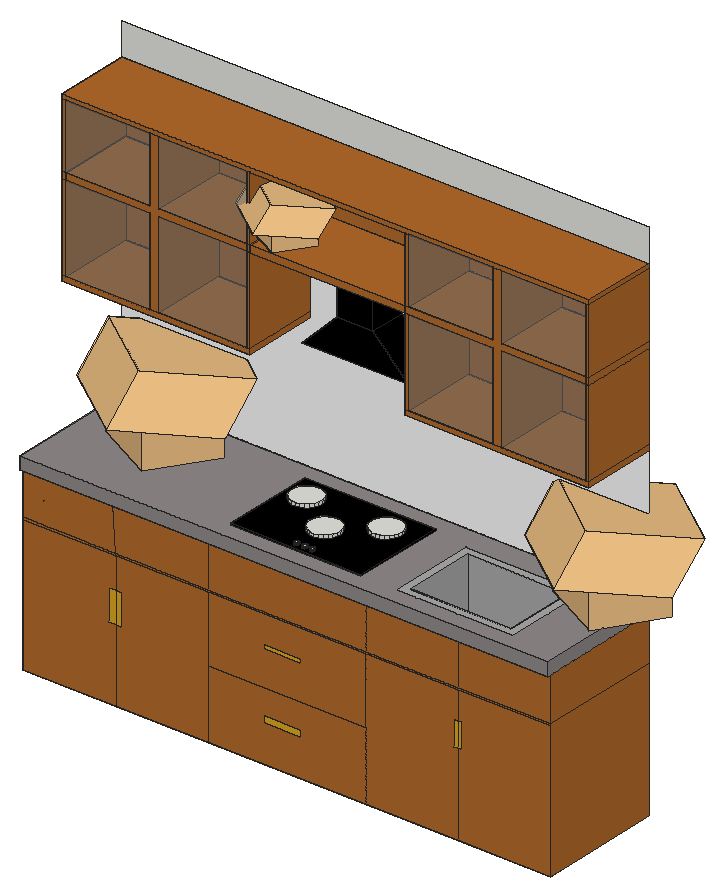
# SketchUp Ruby script. Lengths in inches.
U = 1.inch
M = Sketchup.active_model
def pt(a) = Geom::Point3d.new(a.map { |v| v * U })
def face(e, loops, mat)
  f = e.add_face(loops[0].map { |a| pt(a) })
  loops[1..].each { |l| e.add_face(l.map { |a| pt(a) }).erase! }
  f.material = f.back_material = mat if mat
  f
end
# faces: each face lists its corners as indices into pts; further lists are holes
def faces(e, pts, list, mat = nil) = list.each { |f| face(e, (f[0].is_a?(Array) ? f : [f]).map { |l| l.map { |i| pts[i] } }, mat) }
# xy, xz, yz: faces in a plane at the given z, y or x. An outline is a flat list of corners, or four numbers for a rectangle; further outlines are holes
def ring(l) = l.size == 4 ? [[l[0], l[1]], [l[2], l[1]], [l[2], l[3]], [l[0], l[3]]] : l.each_slice(2).to_a
def flat(e, list, mat, &to3) = list.each { |f| face(e, (f[0].is_a?(Array) ? f : [f]).map { |l| ring(l).map { |u, v| to3.(u, v) } }, mat) }
def xy(e, z, list, mat = nil) = flat(e, list, mat) { |x, y| [x, y, z] }
def xz(e, y, list, mat = nil) = flat(e, list, mat) { |x, z| [x, y, z] }
def yz(e, x, list, mat = nil) = flat(e, list, mat) { |y, z| [x, y, z] }
def lines(e, pts, list) = list.each { |a, b| e.add_line(pt(pts[a]), pt(pts[b])) }
# prism: a flat outline (further loops are holes) pulled along v
def prism(e, loops, v, mat = nil)
  f = face(e, loops, mat); d = Geom::Vector3d.new(v.map { |x| x * U })
  f.pushpull(f.normal.samedirection?(d) ? d.length : -d.length)
end
def box(e, o, s, mat = nil) = prism(e, [[o, [o[0] + s[0], o[1], o[2]], [o[0] + s[0], o[1] + s[1], o[2]], [o[0], o[1] + s[1], o[2]]]], [0, 0, s[2]], mat)
def at(x, y, z, deg = 0) = Geom::Transformation.translation(pt([x, y, z])) * Geom::Transformation.rotation(ORIGIN, Z_AXIS, deg.degrees)
def axes(o, x, y, z) = Geom::Transformation.new([*x, 0, *y, 0, *z, 0, *pt(o).to_a, 1])
def part(name) = M.definitions.add(name)
# library, detail: a bought-in or finely detailed component or shape, given as its bounding box
def library(name, o, s) = part(name).tap { |d| box(d.entities, o, s) }
def detail(e, o, s) = box(e.add_group.entities, o, s)
def put(e, d, t, mat = nil) = e.add_instance(d, t).tap { |i| i.material = mat if mat }
def group(e, t, mat = nil) = e.add_group.tap { |g| g.transformation = t; g.material = mat if mat }.entities
root = M.entities
M.materials.add("Material__1").color = [51, 42, 44]
M.materials.add("Material__2").color = [97, 132, 37]
M.materials.add("[0045_Goldenrod]").color = [218, 165, 32]
M.materials.add("[0129_WhiteSmoke]").color = [245, 245, 245]
M.materials.add("[0132_LightGray]").color = [169, 169, 169]
M.materials.add("[0137_Black]").color = [0, 0, 0]
M.materials.add("[Stone Marble]").color = [143, 138, 136]
M.materials.add("[Translucent Glass Gray]").color = [128, 128, 128]
M.materials["[Translucent Glass Gray]"].alpha = 0.5
M.materials.add("[Wood Bamboo]").color = [177, 105, 43]
c1 = library("\#1",[-138.85,-135.75,0],[277.7,270.97,9.64])
c2 = library("\#2",[-34.84,-73.35,-33.91],[69.68,146.26,68.31])
c3 = library("\#5",[-4127.85,-1300.75,-2324.72],[5349.84,4521.24,5423.31])
c4 = part("\#3")
put(c4.entities,c3,at(450.18,-1111.4375,0),"Material__2")
c5 = part("12")
put(c5.entities,c1,axes([-49.79,-36.9375,349.64],[0.59279,0,0],[0,0.59279,0],[0,0,0.59279]),"Material__1")
put(c5.entities,c2,axes([-39.24,-18.18,177.19],[1.20819,-2.09264,0],[0,0,2.41638],[2.09264,1.20819,0]))
put(c5.entities,c4,axes([-83.44,-46.04,442.44],[-0.03636,-0.03293,-0.01473],[-0.00083,-0.02391,0.05549],[0.02997,-0.02791,-0.01158]))
xy(root,0,[[0,0.8125,120,28.9375]])
xy(root,20,[[84.43,5.43,107.27,21.77]])
xy(root,31.06,[[0,0.8125,120,28.9375]],"[0132_LightGray]")
xy(root,41.12,[[0,0,120,0.8125]])
xy(root,44,[[44.92,3.63,74.67,24.88]])
xy(root,44,[[[82.57,3.57,109.13,23.63],[84.43,5.43,107.27,21.77]]],"[0132_LightGray]")
xy(root,44,[[[0,0,120,28.9375],[44.92,3.63,74.67,24.88],[82.57,3.57,109.13,23.63]]],"[Stone Marble]")
xy(root,44.37,[[58.75,4.66,58.62,4.68,58.5,4.73,58.4,4.81,58.32,4.91,58.27,5.03,58.25,5.16,58.27,5.29,58.32,5.41,58.4,5.52,58.5,5.6,58.62,5.65,58.75,5.66,58.88,5.65,59,5.6,59.1,5.52,59.18,5.41,59.23,5.29,59.25,5.16,59.23,5.03,59.18,4.91,59.1,4.81,59,4.73,58.88,4.68],[60.625,4.66,60.49,4.68,60.375,4.73,60.27,4.81,60.19,4.91,60.14,5.03,60.125,5.16,60.14,5.29,60.19,5.41,60.27,5.52,60.375,5.6,60.49,5.65,60.625,5.66,60.75,5.65,60.875,5.6,60.98,5.52,61.06,5.41,61.11,5.29,61.125,5.16,61.11,5.03,61.06,4.91,60.98,4.81,60.875,4.73,60.75,4.68],[62.375,4.66,62.24,4.68,62.125,4.73,62.02,4.81,61.94,4.91,61.89,5.03,61.875,5.16,61.89,5.29,61.94,5.41,62.02,5.52,62.125,5.6,62.24,5.65,62.375,5.66,62.5,5.65,62.625,5.6,62.73,5.52,62.81,5.41,62.86,5.29,62.875,5.16,62.86,5.03,62.81,4.91,62.73,4.81,62.625,4.73,62.5,4.68],[59.57,9.07,58.68,9.12,57.83,9.4,57.08,9.89,56.48,10.5625,56.08,11.37,55.9,12.24,55.95,13.14,56.23,13.99,56.72,14.74,57.39,15.34,58.2,15.74,59.07,15.92,59.97,15.87,60.82,15.59,61.57,15.09,62.17,14.42,62.57,13.62,62.75,12.74,62.7,11.85,62.42,11,61.93,10.25,61.26,9.65,60.45,9.25],[50.07,15.72,49.17,15.77,48.32,16.06,47.57,16.55,46.97,17.22,46.57,18.02,46.39,18.9,46.44,19.8,46.72,20.65,47.22,21.4,47.89,21.99,48.6875,22.4,49.57,22.58,50.46,22.53,51.31,22.24,52.0625,21.75,52.66,21.08,53.0625,20.28,53.25,19.4,53.19,18.5,52.91,17.65,52.42,16.9,51.75,16.31,50.95,15.9],
  [68.25,15.72,67.36,15.77,66.51,16.06,65.76,16.55,65.16,17.22,64.76,18.02,64.58,18.9,64.63,19.8,64.91,20.65,65.4,21.4,66.07,21.99,66.875,22.4,67.75,22.58,68.65,22.53,69.5,22.24,70.25,21.75,70.85,21.08,71.25,20.28,71.43,19.4,71.38,18.5,71.1,17.65,70.61,16.9,69.93,16.31,69.13,15.9]])
xy(root,44.37,[[[44.92,3.63,74.67,24.88],[50.07,15.72,49.17,15.77,48.32,16.06,47.57,16.55,46.97,17.22,46.57,18.02,46.39,18.9,46.44,19.8,46.72,20.65,47.22,21.4,47.89,21.99,48.6875,22.4,49.57,22.58,50.46,22.53,51.31,22.24,52.0625,21.75,52.66,21.08,53.0625,20.28,53.25,19.4,53.19,18.5,52.91,17.65,52.42,16.9,51.75,16.31,50.95,15.9],[68.25,15.72,67.36,15.77,66.51,16.06,65.76,16.55,65.16,17.22,64.76,18.02,64.58,18.9,64.63,19.8,64.91,20.65,65.4,21.4,66.07,21.99,66.875,22.4,67.75,22.58,68.65,22.53,69.5,22.24,70.25,21.75,70.85,21.08,71.25,20.28,71.43,19.4,71.38,18.5,71.1,17.65,70.61,16.9,69.93,16.31,69.13,15.9],[59.57,9.07,58.68,9.12,57.83,9.4,57.08,9.89,56.48,10.5625,56.08,11.37,55.9,12.24,55.95,13.14,56.23,13.99,56.72,14.74,57.39,15.34,58.2,15.74,59.07,15.92,59.97,15.87,60.82,15.59,61.57,15.09,62.17,14.42,62.57,13.62,62.75,12.74,62.7,11.85,62.42,11,61.93,10.25,61.26,9.65,60.45,9.25],[58.75,4.66,58.62,4.68,58.5,4.73,58.4,4.81,58.32,4.91,58.27,5.03,58.25,5.16,58.27,5.29,58.32,5.41,58.4,5.52,58.5,5.6,58.62,5.65,58.75,5.66,58.88,5.65,59,5.6,59.1,5.52,59.18,5.41,59.23,5.29,59.25,5.16,59.23,5.03,59.18,4.91,59.1,4.81,59,4.73,58.88,4.68],[60.625,4.66,60.49,4.68,60.375,4.73,60.27,4.81,60.19,4.91,60.14,5.03,60.125,5.16,60.14,5.29,60.19,5.41,60.27,5.52,60.375,5.6,60.49,5.65,60.625,5.66,60.75,5.65,60.875,5.6,60.98,5.52,61.06,5.41,61.11,5.29,61.125,5.16,61.11,5.03,61.06,4.91,60.98,4.81,60.875,4.73,60.75,4.68],[62.375,4.66,62.24,4.68,62.125,4.73,62.02,4.81,61.94,4.91,61.89,5.03,61.875,5.16,61.89,5.29,61.94,5.41,62.02,5.52,62.125,5.6,62.24,5.65,62.375,5.66,62.5,5.65,62.625,5.6,62.73,5.52,62.81,5.41,62.86,5.29,62.875,5.16,62.86,5.03,62.81,4.91,62.73,4.81,62.625,4.73,62.5,4.68]]],"[0137_Black]")
xy(root,44.75,[[58.75,4.66,58.88,4.68,59,4.73,59.1,4.81,59.18,4.91,59.23,5.03,59.25,5.16,59.23,5.29,59.18,5.41,59.1,5.52,59,5.6,58.88,5.65,58.75,5.66,58.62,5.65,58.5,5.6,58.4,5.52,58.32,5.41,58.27,5.29,58.25,5.16,58.27,5.03,58.32,4.91,58.4,4.81,58.5,4.73,58.62,4.68],[60.625,4.66,60.75,4.68,60.875,4.73,60.98,4.81,61.06,4.91,61.11,5.03,61.125,5.16,61.11,5.29,61.06,5.41,60.98,5.52,60.875,5.6,60.75,5.65,60.625,5.66,60.49,5.65,60.375,5.6,60.27,5.52,60.19,5.41,60.14,5.29,60.125,5.16,60.14,5.03,60.19,4.91,60.27,4.81,60.375,4.73,60.49,4.68],[62.375,4.66,62.5,4.68,62.625,4.73,62.73,4.81,62.81,4.91,62.86,5.03,62.875,5.16,62.86,5.29,62.81,5.41,62.73,5.52,62.625,5.6,62.5,5.65,62.375,5.66,62.24,5.65,62.125,5.6,62.02,5.52,61.94,5.41,61.89,5.29,61.875,5.16,61.89,5.03,61.94,4.91,62.02,4.81,62.125,4.73,62.24,4.68]])
xy(root,45.06,[[59.57,9.07,60.45,9.25,61.26,9.65,61.93,10.25,62.42,11,62.7,11.85,62.75,12.74,62.57,13.62,62.17,14.42,61.57,15.09,60.82,15.59,59.97,15.87,59.07,15.92,58.2,15.74,57.39,15.34,56.72,14.74,56.23,13.99,55.95,13.14,55.9,12.24,56.08,11.37,56.48,10.5625,57.08,9.89,57.83,9.4,58.68,9.12],[50.07,15.72,50.95,15.9,51.75,16.31,52.42,16.9,52.91,17.65,53.19,18.5,53.25,19.4,53.0625,20.28,52.66,21.08,52.0625,21.75,51.31,22.24,50.46,22.53,49.57,22.58,48.6875,22.4,47.89,21.99,47.22,21.4,46.72,20.65,46.44,19.8,46.39,18.9,46.57,18.02,46.97,17.22,47.57,16.55,48.32,16.06,49.17,15.77],[68.25,15.72,69.13,15.9,69.93,16.31,70.61,16.9,71.1,17.65,71.38,18.5,71.43,19.4,71.25,20.28,70.85,21.08,70.25,21.75,69.5,22.24,68.65,22.53,67.75,22.58,66.875,22.4,66.07,21.99,65.4,21.4,64.91,20.65,64.63,19.8,64.58,18.9,64.76,18.02,65.16,17.22,65.76,16.55,66.51,16.06,67.36,15.77]])
xy(root,74.4,[[0,11.875,42.84,28.9375],[78,11.875,120,28.9375]],"[Wood Bamboo]")
xy(root,74.65,[[47.6,20.6875,71.54,28.9375]],"[0137_Black]")
xy(root,75.5625,[[0,11.875,0.85,28.9375],[20,11.875,22,28.9375],[42,11.875,42.84,28.9375],[78,11.875,78.84,28.9375],[98,11.875,100,28.9375],
  [119.15,11.875,120,28.9375]])
xy(root,75.5625,[[0.85,11.875,20,28.9375],[22,11.875,42,28.9375],[78.84,11.875,98,28.9375],[100,11.875,119.15,28.9375]],"[Wood Bamboo]")
xy(root,82.63,[[55.52,20.6875,63.77,28.9375]])
xy(root,95.2,[[55.52,20.6875,63.77,28.9375]])
xy(root,95.2,[[0,11.875,20,28.9375],[22,11.875,42,28.9375],[42,11.875,42,28.9375,55.52,28.9375,55.52,20.6875,63.77,20.6875,63.77,28.9375,78,28.9375,78,11.875],[78.84,11.875,98,28.9375],[100,11.875,120,28.9375]],"[Wood Bamboo]")
xy(root,96.71,[[0,11.875,0.85,28.9375],[78,11.875,78.84,28.9375]])
xy(root,96.71,[[0.85,11.875,20,28.9375],[22,11.875,42,28.9375],[42.84,11.875,78,28.9375],[78.84,11.875,98,28.9375],[100,11.875,119.15,28.9375]],"[Wood Bamboo]")
xy(root,111.5625,[[0,11.875,0.85,28.9375],[20,11.875,22,28.9375],[42,11.875,42.84,28.9375],[78,11.875,78.84,28.9375],[98,11.875,100,28.9375],
  [119.15,11.875,120,28.9375]])
xy(root,111.5625,[[0.85,11.875,20,28.9375],[22,11.875,42,28.9375],[42.84,11.875,78,28.9375],[78.84,11.875,98,28.9375],[100,11.875,119.15,28.9375]],"[Wood Bamboo]")
xy(root,112.59,[[0,11.875,120,28.9375]],"[Wood Bamboo]")
xz(root,0,[[0,41.12,120,44]],"[Stone Marble]")
xz(root,0.8125,[[54.6875,8.32,63.25,9.89],[19.625,16.53,21,23.65],[21,16.53,22.5625,23.65],[97.9375,18.72,99,24.4],[99,18.72,99.8125,24.4],
  [54.6875,23.34,63.25,24.4],[4.75,36.15,11.56,37.09],[27.85,36.15,33.97,37.09],[54.6875,36.15,63.25,37.09],[85.85,36.15,91.48,37.09],
  [107.99,36.15,113.12,37.09]],"[0045_Goldenrod]")
xz(root,0.8125,[[0,0,21,0,21,16.53,19.625,16.53,19.625,23.65,21,23.65,21,30.625,0,30.625],[21,0,42,0,42,30.625,21,30.625,21,23.65,22.5625,23.65,22.5625,16.53,21,16.53],[[42,0,78,15.5],[54.6875,8.32,63.25,9.89]],[78,0,99,0,99,18.72,97.9375,18.72,97.9375,24.4,99,24.4,99,30.625,78,30.625],[99,0,120,0,120,30.625,99,30.625,99,24.4,99.8125,24.4,99.8125,18.72,99,18.72],
  [[42,15.5,78,30.625],[54.6875,23.34,63.25,24.4]],[0,30.625,42,31.06],[42,30.625,78,31.06],[78,30.625,99,31.06],[99,30.625,120,31.06],
  [0,31.06,42,41.12],[42,31.06,78,41.12],[78,31.06,99,41.12],[99,31.06,120,41.12]],"[Wood Bamboo]")
xz(root,3.63,[[44.92,44,74.67,44.37]],"[0137_Black]")
xz(root,5.43,[[84.43,20,107.27,44]],"[0132_LightGray]")
xz(root,11.875,[[0.85,75.5625,20,95.2],[22,75.5625,42,95.2],[78.84,75.5625,98,95.2],[100,75.5625,119.15,95.2],[0.85,96.71,20,111.5625],
  [22,96.71,42,111.5625],[78.84,96.71,98,111.5625],[100,96.71,119.15,111.5625]],"[Translucent Glass Gray]")
xz(root,11.875,[[0,74.4,42.84,75.5625],[78,74.4,120,75.5625],[0,75.5625,0.85,95.2],[20,75.5625,22,75.5625,22,95.2,42,95.2,42,96.71,22,96.71,22,111.5625,20,111.5625,20,96.71,0.85,96.71,0.85,95.2,20,95.2],[42,75.5625,42.84,95.2],
  [78,75.5625,78.84,95.2],[98,75.5625,100,75.5625,100,95.2,119.15,95.2,119.15,96.71,100,96.71,100,111.5625,98,111.5625,98,96.71,78,96.71,78,95.2,98,95.2],[119.15,75.5625,120,95.2],[0,95.2,0.85,96.71],[42,95.2,42.84,96.71],
  [42.84,95.2,78,96.71],[119.15,95.2,120,96.71],[0,96.71,0.85,111.5625],[42,96.71,42.84,111.5625],[78,96.71,78.84,111.5625],
  [119.15,96.71,120,111.5625],[0,111.5625,120,112.59]],"[Wood Bamboo]")
xz(root,20.6875,[[47.6,74.65,71.54,74.65,63.77,82.63,55.52,82.63],[55.52,82.63,63.77,95.2]],"[0137_Black]")
xz(root,21.77,[[84.43,20,107.27,44]],"[0132_LightGray]")
xz(root,24.88,[[44.92,44,74.67,44.37]],"[0137_Black]")
xz(root,28.9375,[[0,0,120,31.06],[0,31.06,120,44],[0,74.4,42.84,75.5625],[78,74.4,120,75.5625],[47.6,74.65,55.52,82.63,63.77,82.63,71.54,74.65],
  [0,75.5625,0.85,95.2],[20,75.5625,20,95.2,0.85,95.2,0.85,96.71,20,96.71,20,111.5625,22,111.5625,22,96.71,42,96.71,42,95.2,22,95.2,22,75.5625],[42,75.5625,42.84,95.2],[78,75.5625,78.84,95.2],[98,75.5625,98,95.2,78,95.2,78,96.71,98,96.71,98,111.5625,100,111.5625,100,96.71,119.15,96.71,119.15,95.2,100,95.2,100,75.5625],
  [119.15,75.5625,120,95.2],[55.52,82.63,63.77,95.2],[0,95.2,0.85,96.71],[42,95.2,42.84,96.71],[42.84,95.2,78,96.71],
  [119.15,95.2,120,96.71],[0,96.71,0.85,111.5625],[42,96.71,42.84,111.5625],[78,96.71,78.84,111.5625],[119.15,96.71,120,111.5625],
  [0,111.5625,120,112.59],[0,112.59,120,120]])
xz(root,28.9375,[[0,44,0,74.4,42.84,74.4,42.84,95.2,55.52,95.2,55.52,82.63,47.6,74.65,71.54,74.65,63.77,82.63,63.77,95.2,78,95.2,78,74.4,120,74.4,120,44]],"[0129_WhiteSmoke]")
xz(root,28.9375,[[0.85,75.5625,20,95.2],[22,75.5625,42,95.2],[78.84,75.5625,98,95.2],[100,75.5625,119.15,95.2],[0.85,96.71,20,111.5625],
  [22,96.71,42,111.5625],[42.84,96.71,78,111.5625],[78.84,96.71,98,111.5625],[100,96.71,119.15,111.5625]],"[Wood Bamboo]")
yz(root,0,[[0,41.12,28.9375,44]],"[Stone Marble]")
yz(root,0,[[0.8125,0,28.9375,31.06],[0.8125,31.06,28.9375,41.12],[11.875,74.4,28.9375,75.5625],[11.875,75.5625,28.9375,95.2],[11.875,95.2,28.9375,96.71],
  [11.875,96.71,28.9375,111.5625],[11.875,111.5625,28.9375,112.59]],"[Wood Bamboo]")
yz(root,0.85,[[11.875,75.5625,28.9375,96.71],[11.875,96.71,28.9375,111.5625]],"[Wood Bamboo]")
yz(root,20,[[11.875,75.5625,28.9375,95.2],[11.875,96.71,28.9375,111.5625]],"[Wood Bamboo]")
yz(root,22,[[11.875,75.5625,28.9375,95.2],[11.875,96.71,28.9375,111.5625]],"[Wood Bamboo]")
yz(root,42,[[11.875,95.2,28.9375,96.71]])
yz(root,42,[[11.875,75.5625,28.9375,95.2],[11.875,96.71,28.9375,111.5625]],"[Wood Bamboo]")
yz(root,42.84,[[11.875,74.4,28.9375,75.5625],[11.875,75.5625,28.9375,96.71],[11.875,96.71,28.9375,111.5625]],"[Wood Bamboo]")
yz(root,44.92,[[3.63,44,24.88,44.37]],"[0137_Black]")
yz(root,55.52,[[20.6875,82.63,28.9375,95.2]],"[0137_Black]")
yz(root,63.77,[[20.6875,82.63,28.9375,95.2]],"[0137_Black]")
yz(root,74.67,[[3.63,44,24.88,44.37]],"[0137_Black]")
yz(root,78,[[11.875,95.2,28.9375,96.71]])
yz(root,78,[[11.875,74.4,28.9375,75.5625],[11.875,75.5625,28.9375,95.2],[11.875,96.71,28.9375,111.5625]],"[Wood Bamboo]")
yz(root,78.84,[[11.875,75.5625,28.9375,95.2],[11.875,96.71,28.9375,111.5625]],"[Wood Bamboo]")
yz(root,84.43,[[5.43,20,21.77,44]],"[0132_LightGray]")
yz(root,98,[[11.875,75.5625,28.9375,95.2],[11.875,96.71,28.9375,111.5625]],"[Wood Bamboo]")
yz(root,100,[[11.875,75.5625,28.9375,95.2],[11.875,96.71,28.9375,111.5625]],"[Wood Bamboo]")
yz(root,107.27,[[5.43,20,21.77,44]],"[0132_LightGray]")
yz(root,119.15,[[11.875,75.5625,28.9375,96.71],[11.875,96.71,28.9375,111.5625]],"[Wood Bamboo]")
yz(root,120,[[0,41.12,28.9375,44]],"[Stone Marble]")
yz(root,120,[[0.8125,0,28.9375,31.06],[0.8125,31.06,28.9375,41.12],[11.875,74.4,28.9375,75.5625],[11.875,75.5625,28.9375,95.2],[11.875,95.2,28.9375,96.71],
  [11.875,96.71,28.9375,111.5625],[11.875,111.5625,28.9375,112.59]],"[Wood Bamboo]")
p = [[58.4,4.81,44.37],[58.5,4.73,44.37],[58.5,4.73,44.75],[58.4,4.81,44.75],[58.62,4.68,44.37],[58.62,4.68,44.75],
  [58.75,4.66,44.37],[58.75,4.66,44.75],[58.88,4.68,44.37],[58.88,4.68,44.75],[59,4.73,44.37],[59,4.73,44.75],
  [59.1,4.81,44.37],[59.1,4.81,44.75],[60.27,4.81,44.37],[60.375,4.73,44.37],[60.375,4.73,44.75],[60.27,4.81,44.75],
  [60.49,4.68,44.37],[60.49,4.68,44.75],[60.625,4.66,44.37],[60.625,4.66,44.75],[60.75,4.68,44.37],[60.75,4.68,44.75],
  [60.875,4.73,44.37],[60.875,4.73,44.75],[60.98,4.81,44.37],[60.98,4.81,44.75],[62.02,4.81,44.37],[62.125,4.73,44.37],
  [62.125,4.73,44.75],[62.02,4.81,44.75],[62.24,4.68,44.37],[62.24,4.68,44.75],[62.375,4.66,44.37],[62.375,4.66,44.75],
  [62.5,4.68,44.37],[62.5,4.68,44.75],[62.625,4.73,44.37],[62.625,4.73,44.75],[62.73,4.81,44.37],[62.73,4.81,44.75],
  [58.32,4.91,44.37],[58.32,4.91,44.75],[59.18,4.91,44.37],[59.18,4.91,44.75],[60.19,4.91,44.37],[60.19,4.91,44.75],
  [61.06,4.91,44.37],[61.06,4.91,44.75],[61.94,4.91,44.37],[61.94,4.91,44.75],[62.81,4.91,44.37],[62.81,4.91,44.75],
  [58.27,5.03,44.37],[58.27,5.03,44.75],[59.23,5.03,44.37],[59.23,5.03,44.75],[60.14,5.03,44.37],[60.14,5.03,44.75],
  [61.11,5.03,44.37],[61.11,5.03,44.75],[61.89,5.03,44.37],[61.89,5.03,44.75],[62.86,5.03,44.37],[62.86,5.03,44.75],
  [58.25,5.16,44.37],[58.25,5.16,44.75],[59.25,5.16,44.37],[59.25,5.16,44.75],[60.125,5.16,44.37],[60.125,5.16,44.75],
  [61.125,5.16,44.37],[61.125,5.16,44.75],[61.875,5.16,44.37],[61.875,5.16,44.75],[62.875,5.16,44.37],[62.875,5.16,44.75],
  [58.27,5.29,44.37],[58.27,5.29,44.75],[59.23,5.29,44.37],[59.23,5.29,44.75],[60.14,5.29,44.37],[60.14,5.29,44.75],
  [61.11,5.29,44.37],[61.11,5.29,44.75],[61.89,5.29,44.37],[61.89,5.29,44.75],[62.86,5.29,44.37],[62.86,5.29,44.75],
  [58.32,5.41,44.37],[58.32,5.41,44.75],[59.18,5.41,44.37],[59.18,5.41,44.75],[60.19,5.41,44.37],[60.19,5.41,44.75],
  [61.06,5.41,44.37],[61.06,5.41,44.75],[61.94,5.41,44.37],[61.94,5.41,44.75],[62.81,5.41,44.37],[62.81,5.41,44.75],
  [58.4,5.52,44.37],[58.4,5.52,44.75],[59.1,5.52,44.37],[59.1,5.52,44.75],[60.27,5.52,44.37],[60.27,5.52,44.75],
  [60.98,5.52,44.37],[60.98,5.52,44.75],[62.02,5.52,44.37],[62.02,5.52,44.75],[62.73,5.52,44.37],[62.73,5.52,44.75],
  [58.5,5.6,44.37],[58.5,5.6,44.75],[59,5.6,44.37],[59,5.6,44.75],[60.375,5.6,44.37],[60.375,5.6,44.75],
  [60.875,5.6,44.37],[60.875,5.6,44.75],[62.125,5.6,44.37],[62.125,5.6,44.75],[62.625,5.6,44.37],[62.625,5.6,44.75],
  [58.62,5.65,44.37],[58.62,5.65,44.75],[58.75,5.66,44.37],[58.75,5.66,44.75],[58.88,5.65,44.37],[58.88,5.65,44.75],
  [60.49,5.65,44.37],[60.49,5.65,44.75],[60.625,5.66,44.37],[60.625,5.66,44.75],[60.75,5.65,44.37],[60.75,5.65,44.75],
  [62.24,5.65,44.37],[62.24,5.65,44.75],[62.375,5.66,44.37],[62.375,5.66,44.75],[62.5,5.65,44.37],[62.5,5.65,44.75],
  [57.83,9.4,44.37],[58.68,9.12,44.37],[58.68,9.12,45.06],[57.83,9.4,45.06],[59.57,9.07,44.37],[59.57,9.07,45.06],
  [60.45,9.25,44.37],[60.45,9.25,45.06],[61.26,9.65,44.37],[61.26,9.65,45.06],[57.08,9.89,44.37],[57.08,9.89,45.06],
  [61.93,10.25,44.37],[61.93,10.25,45.06],[56.48,10.5625,44.37],[56.48,10.5625,45.06],[62.42,11,44.37],[62.42,11,45.06],
  [56.08,11.37,44.37],[56.08,11.37,45.06],[62.7,11.85,44.37],[62.7,11.85,45.06],[55.9,12.24,44.37],[55.9,12.24,45.06],
  [62.75,12.74,44.37],[62.75,12.74,45.06],[55.95,13.14,44.37],[55.95,13.14,45.06],[62.57,13.62,44.37],[62.57,13.62,45.06],
  [56.23,13.99,44.37],[56.23,13.99,45.06],[62.17,14.42,44.37],[62.17,14.42,45.06],[56.72,14.74,44.37],[56.72,14.74,45.06],
  [61.57,15.09,44.37],[61.57,15.09,45.06],[57.39,15.34,44.37],[57.39,15.34,45.06],[60.82,15.59,44.37],[60.82,15.59,45.06],
  [58.2,15.74,44.37],[58.2,15.74,45.06],[59.97,15.87,44.37],[59.97,15.87,45.06],[49.17,15.77,44.37],[50.07,15.72,44.37],
  [50.07,15.72,45.06],[49.17,15.77,45.06],[50.95,15.9,44.37],[50.95,15.9,45.06],[59.07,15.92,44.37],[59.07,15.92,45.06],
  [67.36,15.77,44.37],[68.25,15.72,44.37],[68.25,15.72,45.06],[67.36,15.77,45.06],[69.13,15.9,44.37],[69.13,15.9,45.06],
  [48.32,16.06,44.37],[48.32,16.06,45.06],[66.51,16.06,44.37],[66.51,16.06,45.06],[51.75,16.31,44.37],[51.75,16.31,45.06],
  [69.93,16.31,44.37],[69.93,16.31,45.06],[47.57,16.55,44.37],[47.57,16.55,45.06],[65.76,16.55,44.37],[65.76,16.55,45.06],
  [52.42,16.9,44.37],[52.42,16.9,45.06],[70.61,16.9,44.37],[70.61,16.9,45.06],[46.97,17.22,44.37],[46.97,17.22,45.06],
  [65.16,17.22,44.37],[65.16,17.22,45.06],[52.91,17.65,44.37],[52.91,17.65,45.06],[71.1,17.65,44.37],[71.1,17.65,45.06],
  [46.57,18.02,44.37],[46.57,18.02,45.06],[64.76,18.02,44.37],[64.76,18.02,45.06],[53.19,18.5,44.37],[53.19,18.5,45.06],
  [71.38,18.5,44.37],[71.38,18.5,45.06],[46.39,18.9,44.37],[46.39,18.9,45.06],[64.58,18.9,44.37],[64.58,18.9,45.06],
  [53.25,19.4,44.37],[53.25,19.4,45.06],[71.43,19.4,44.37],[71.43,19.4,45.06],[46.44,19.8,44.37],[46.44,19.8,45.06],
  [64.63,19.8,44.37],[64.63,19.8,45.06],[53.0625,20.28,44.37],[53.0625,20.28,45.06],[71.25,20.28,44.37],[71.25,20.28,45.06],
  [46.72,20.65,44.37],[46.72,20.65,45.06],[64.91,20.65,44.37],[64.91,20.65,45.06],[52.66,21.08,44.37],[52.66,21.08,45.06],
  [70.85,21.08,44.37],[70.85,21.08,45.06],[47.22,21.4,44.37],[47.22,21.4,45.06],[65.4,21.4,44.37],[65.4,21.4,45.06],
  [52.0625,21.75,44.37],[52.0625,21.75,45.06],[70.25,21.75,44.37],[70.25,21.75,45.06],[47.89,21.99,44.37],[47.89,21.99,45.06],
  [66.07,21.99,44.37],[66.07,21.99,45.06],[51.31,22.24,44.37],[51.31,22.24,45.06],[69.5,22.24,44.37],[69.5,22.24,45.06],
  [48.6875,22.4,44.37],[48.6875,22.4,45.06],[66.875,22.4,44.37],[66.875,22.4,45.06],[50.46,22.53,44.37],[50.46,22.53,45.06],
  [68.65,22.53,44.37],[68.65,22.53,45.06],[49.57,22.58,44.37],[49.57,22.58,45.06],[67.75,22.58,44.37],[67.75,22.58,45.06],
  [55.52,28.9375,82.63],[47.6,28.9375,74.65],[47.6,20.6875,74.65],[55.52,20.6875,82.63],[71.54,28.9375,74.65],[63.77,28.9375,82.63],
  [63.77,20.6875,82.63],[71.54,20.6875,74.65],[21,0,41.12],[21,0.8125,30.625]]
faces(root,p,[[0,1,2,3],[1,4,5,2],[4,6,7,5],[6,8,9,7],[8,10,11,9],[10,12,13,11],[14,15,16,17],[15,18,19,16],
  [18,20,21,19],[20,22,23,21],[22,24,25,23],[24,26,27,25],[28,29,30,31],[29,32,33,30],[32,34,35,33],[34,36,37,35],
  [36,38,39,37],[38,40,41,39],[42,0,3,43],[12,44,45,13],[46,14,17,47],[26,48,49,27],[50,28,31,51],[40,52,53,41],
  [54,42,43,55],[44,56,57,45],[58,46,47,59],[48,60,61,49],[62,50,51,63],[52,64,65,53],[66,54,55,67],[56,68,69,57],
  [70,58,59,71],[60,72,73,61],[74,62,63,75],[64,76,77,65],[78,66,67,79],[68,80,81,69],[82,70,71,83],[72,84,85,73],
  [86,74,75,87],[76,88,89,77],[90,78,79,91],[80,92,93,81],[94,82,83,95],[84,96,97,85],[98,86,87,99],[88,100,101,89],
  [102,90,91,103],[92,104,105,93],[106,94,95,107],[96,108,109,97],[110,98,99,111],[100,112,113,101],[114,102,103,115],[104,116,117,105],
  [118,106,107,119],[108,120,121,109],[122,110,111,123],[112,124,125,113],[126,114,115,127],[128,126,127,129],[130,128,129,131],[116,130,131,117],
  [132,118,119,133],[134,132,133,135],[136,134,135,137],[120,136,137,121],[138,122,123,139],[140,138,139,141],[142,140,141,143],[124,142,143,125],
  [144,145,146,147],[145,148,149,146],[148,150,151,149],[150,152,153,151],[154,144,147,155],[152,156,157,153],[158,154,155,159],[156,160,161,157],
  [162,158,159,163],[160,164,165,161],[166,162,163,167],[164,168,169,165],[170,166,167,171],[168,172,173,169],[174,170,171,175],[172,176,177,173],
  [178,174,175,179],[176,180,181,177],[182,178,179,183],[180,184,185,181],[186,182,183,187],[184,188,189,185],[190,191,192,193],[191,194,195,192],
  [196,186,187,197],[198,199,200,201],[199,202,203,200],[204,190,193,205],[206,198,201,207],[194,208,209,195],[188,196,197,189],[202,210,211,203],
  [212,204,205,213],[214,206,207,215],[208,216,217,209],[210,218,219,211],[220,212,213,221],[222,214,215,223],[216,224,225,217],[218,226,227,219],
  [228,220,221,229],[230,222,223,231],[224,232,233,225],[226,234,235,227],[236,228,229,237],[238,230,231,239],[232,240,241,233],[234,242,243,235],
  [244,236,237,245],[246,238,239,247],[240,248,249,241],[242,250,251,243],[252,244,245,253],[254,246,247,255],[248,256,257,249],[250,258,259,251],
  [260,252,253,261],[262,254,255,263],[256,264,265,257],[258,266,267,259],[268,260,261,269],[270,262,263,271],[264,272,273,265],[266,274,275,267],
  [276,268,269,277],[278,270,271,279],[272,280,281,273],[274,282,283,275],[284,276,277,285],[286,278,279,287],[280,284,285,281],[282,286,287,283]])
faces(root,p,[[288,289,290,291],[292,293,294,295]],"[0137_Black]")
lines(root,p,[[296,297]])
put(root,c5,axes([50.69,13.63,99.04],[0.05489,0,0],[0,-0.04861,0],[0,0,0.01468]))
put(root,c5,axes([21.35,17.61,44],[0.099,0,0],[0,-0.0891,0],[0,0,0.03086]))
put(root,c5,axes([119.56,22.16,44],[0.099,0,0],[0,-0.0891,0],[0,0,0.03086]))
